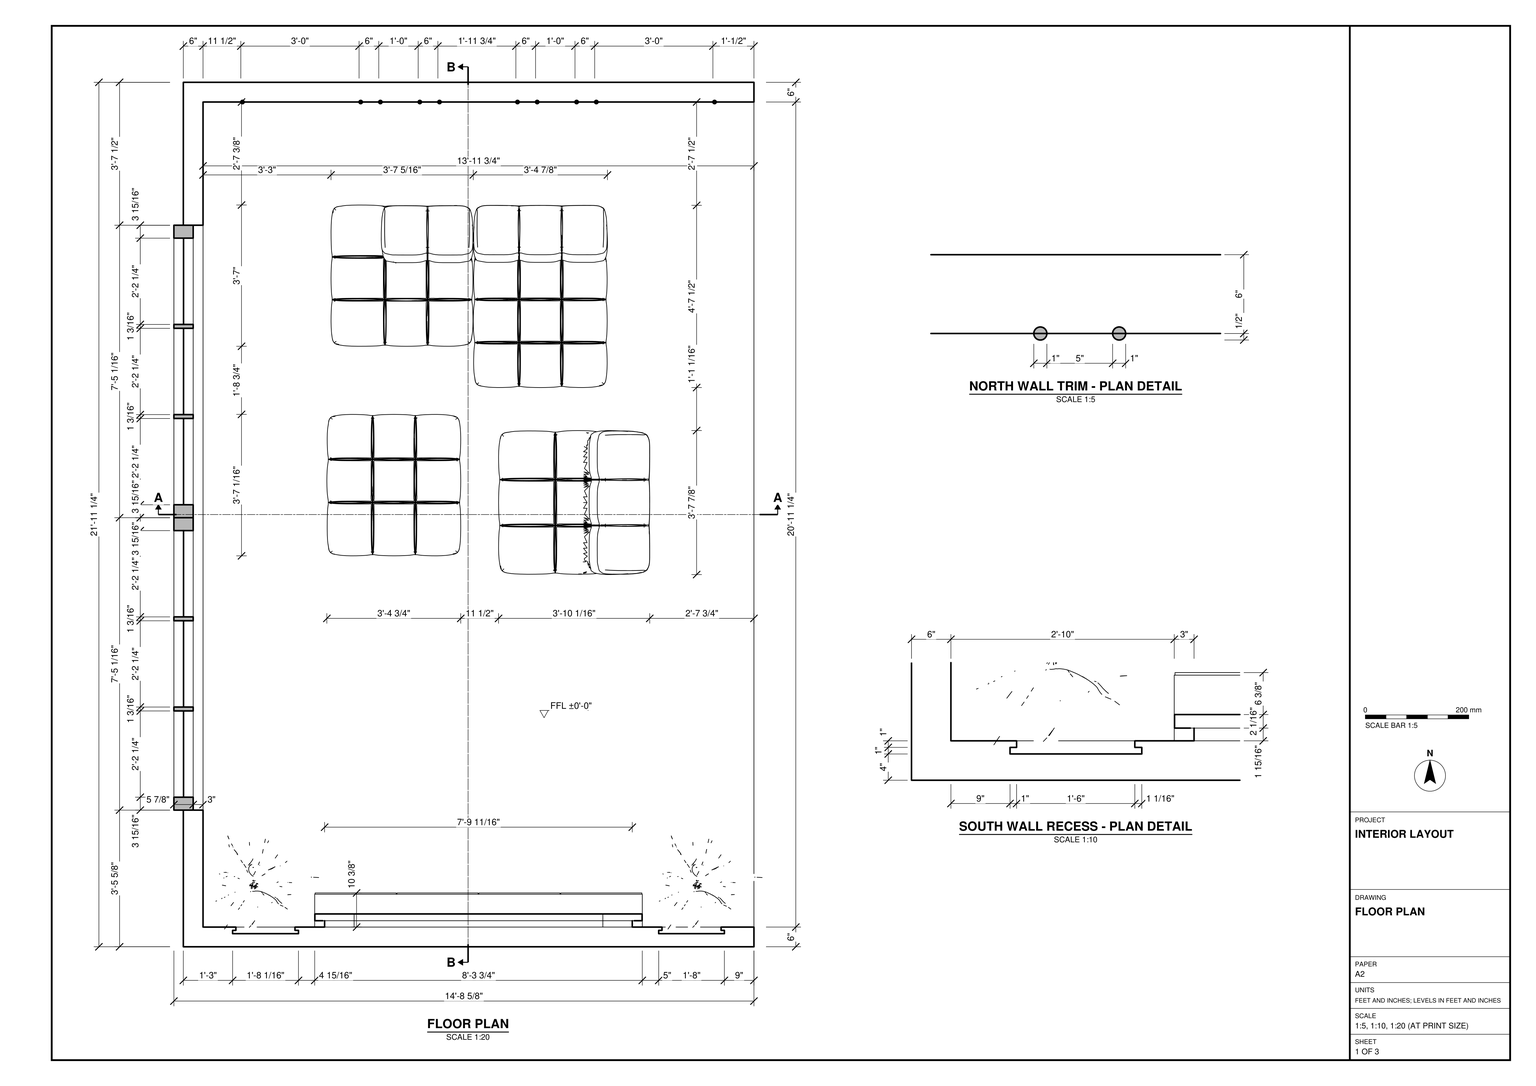
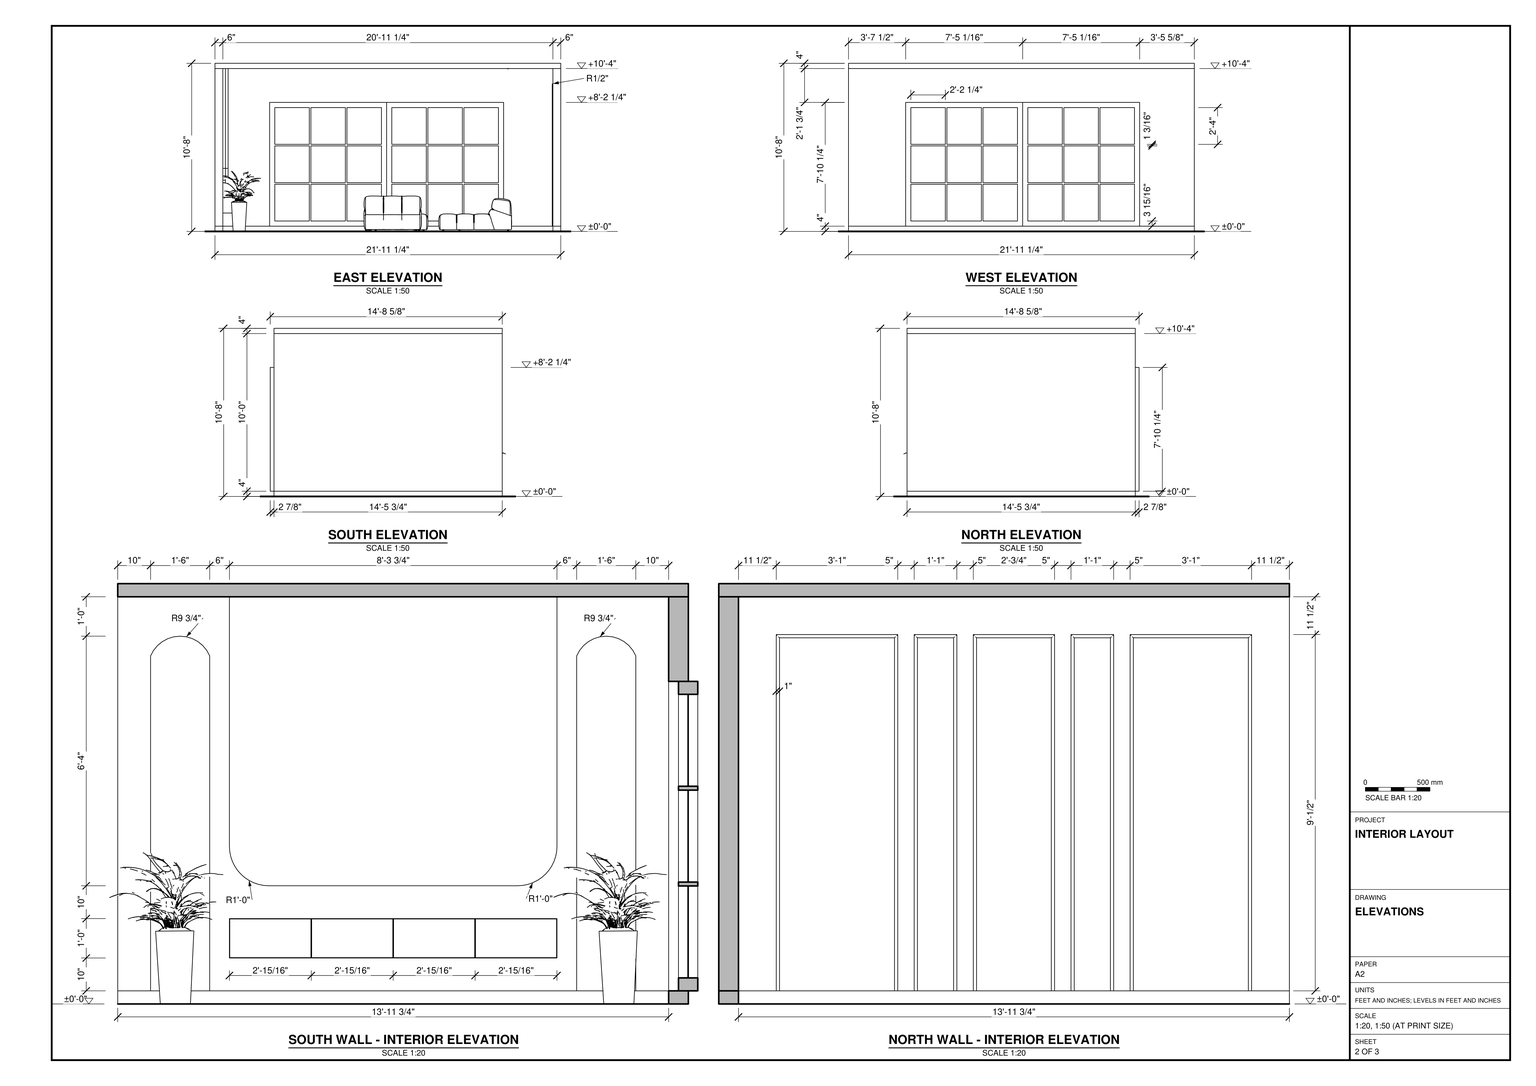
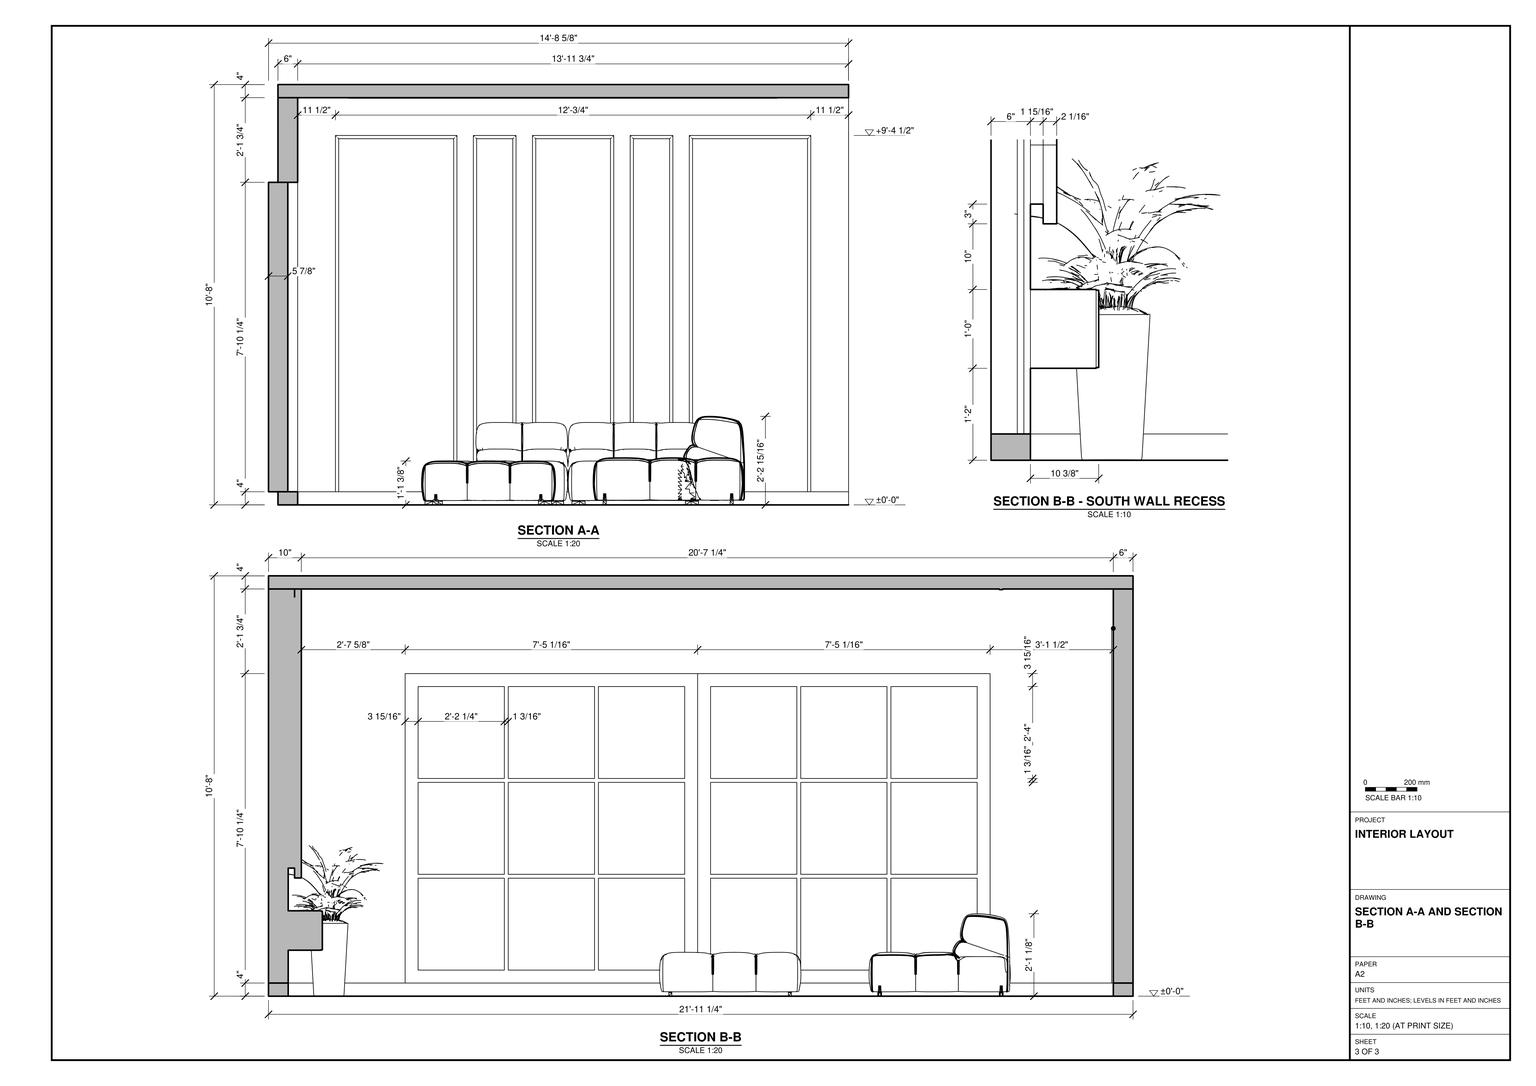
Build the lounge in SketchUp from task_files/diagram_01.pdf. Work in feet and inches. Use the floor plan to orient the room, with north at the top. The overall model extents are 14'-11 3/16" east to west, 21'-11 1/4" north to south and 10'-8" high. Use ±0'-0" as the single floor level.

Model the floor and ceiling slabs and the north, south and west walls with the thicknesses shown in plan and section. Leave the east side open as drawn. Fit the paired window units into the west wall, matching their frames and pane divisions. On the north wall, reproduce the tall rectangular trim outlines in their alternating widths. On the south wall, form the central panel with rounded lower corners, the arched recesses on either side and the floating four-front cabinet below the panel. Use the detail views to distinguish the recessed features from the projecting joinery.

Arrange the modular sofa toward the north wall with its deeper section on the east. Place the separate ottoman and backed seat to its south, matching their footprints and the gap between them. Decor and loose items, including the plants flanking the cabinet, may be any suitable library components, for example from 3D Warehouse. Keep shell elements and each furniture or joinery piece in separate groups or components, and use components for repeated parts. Save one SketchUp model as output_files/lounge_with_modular_seating_and_fitted_feature_walls.skp.

# SketchUp Ruby script. Lengths in inches.
U = 1.inch
M = Sketchup.active_model
def pt(a) = Geom::Point3d.new(a.map { |v| v * U })
def face(e, loops, mat)
  f = e.add_face(loops[0].map { |a| pt(a) })
  loops[1..].each { |l| e.add_face(l.map { |a| pt(a) }).erase! }
  f.material = f.back_material = mat if mat
  f
end
# faces: each face lists its corners as indices into pts; further lists are holes
def faces(e, pts, list, mat = nil) = list.each { |f| face(e, (f[0].is_a?(Array) ? f : [f]).map { |l| l.map { |i| pts[i] } }, mat) }
# xy, xz, yz: faces in a plane at the given z, y or x. An outline is a flat list of corners, or four numbers for a rectangle; further outlines are holes
def ring(l) = l.size == 4 ? [[l[0], l[1]], [l[2], l[1]], [l[2], l[3]], [l[0], l[3]]] : l.each_slice(2).to_a
def flat(e, list, mat, &to3) = list.each { |f| face(e, (f[0].is_a?(Array) ? f : [f]).map { |l| ring(l).map { |u, v| to3.(u, v) } }, mat) }
def xy(e, z, list, mat = nil) = flat(e, list, mat) { |x, y| [x, y, z] }
def xz(e, y, list, mat = nil) = flat(e, list, mat) { |x, z| [x, y, z] }
def yz(e, x, list, mat = nil) = flat(e, list, mat) { |y, z| [x, y, z] }
def lines(e, pts, list) = list.each { |a, b| e.add_line(pt(pts[a]), pt(pts[b])) }
# prism: a flat outline (further loops are holes) pulled along v
def prism(e, loops, v, mat = nil)
  f = face(e, loops, mat); d = Geom::Vector3d.new(v.map { |x| x * U })
  f.pushpull(f.normal.samedirection?(d) ? d.length : -d.length)
end
def box(e, o, s, mat = nil) = prism(e, [[o, [o[0] + s[0], o[1], o[2]], [o[0] + s[0], o[1] + s[1], o[2]], [o[0], o[1] + s[1], o[2]]]], [0, 0, s[2]], mat)
def at(x, y, z, deg = 0) = Geom::Transformation.translation(pt([x, y, z])) * Geom::Transformation.rotation(ORIGIN, Z_AXIS, deg.degrees)
def axes(o, x, y, z) = Geom::Transformation.new([*x, 0, *y, 0, *z, 0, *pt(o).to_a, 1])
def part(name) = M.definitions.add(name)
# library, detail: a bought-in or finely detailed component or shape, given as its bounding box
def library(name, o, s) = part(name).tap { |d| box(d.entities, o, s) }
def detail(e, o, s) = box(e.add_group.entities, o, s)
def put(e, d, t, mat = nil) = e.add_instance(d, t).tap { |i| i.material = mat if mat }
def group(e, t, mat = nil) = e.add_group.tap { |g| g.transformation = t; g.material = mat if mat }.entities
root = M.entities
M.materials.add("Emissive").color = [255, 255, 255]
M.materials.add("Generic").color = [218, 212, 201]
M.materials.add("Pine Matte 300cm").color = [173, 150, 115]
M.materials.add("Sandstone 150cm").color = [161, 146, 124]
M.materials.add("Stucco Shadow 300cm").color = [61, 59, 79]
M.materials.add("Sumele_Hair").color = [19, 13, 7]
M.materials.add("WALL P 1").color = [209, 201, 189]
M.materials.add("WALL P 2").color = [44, 39, 31]
M.materials.add("Wall Paint Dusk Blue Matte 300cm").color = [122, 143, 157]
M.materials.add("Wall Paint Olive Satin 300cm").color = [133, 140, 86]
M.materials.add("Wallpaper A04 Golden 40cm").color = [81, 64, 34]
M.materials.add("Walnut Matte 300cm").color = [111, 85, 55]
M.materials.add("[Metal Corrugated Shiny]").color = [193, 193, 193]
M.materials.add("[Translucent Glass Gray]").color = [128, 128, 128]
M.materials["[Translucent Glass Gray]"].alpha = 0.5
M.materials.add("sofa .").color = [225, 194, 69]
c1 = library("skpD0I6a8",[14.43,-68.68,0],[105.42,143.14,64.75])
c2 = library("skpcyxm1p",[14.43,-75.28,0],[105.19,111.11,34.48])
c3 = library("Modular lounge seating",[0,0,0],[105.41,111.76,64.75])
c4 = library("skp0QfVtK",[14.45,-36.06,-0.05],[111.77,111,64.8])
c5 = library("IES Light",[-4.45,-4.45,-12],[8.9,8.9,12])
c6 = part("Group30\#1")
p = [[0,0,0],[0,0,-64.71],[-12.88,0,-64.71],[83.875,-125.625,0],[-83.875,-125.625,0],[83.875,125.625,0],
  [83.875,0,0],[-83.875,125.625,0],[12.88,0,-64.71],[-83.875,0,0],[0,0,-104.75]]
lines(c6.entities,p,[[0,1],[1,2],[3,4],[5,6],[7,5],[1,8],[9,0],[0,6],[8,10],[4,9],[6,3],[2,10],
  [9,7]])
c7 = part("Rectangle Light")
put(c7.entities,c6,at(0,0,0))
c8 = library("Plant",[-15.17,-14.95,0],[35.27,31.45,46.14])
c9 = part("Group2\#2")
xy(c9.entities,0,[[-40.59,-43.18,-14.32,-15.18],[-13.13,-43.18,13.13,-15.18],[14.32,-43.18,40.59,-15.18],[-40.59,-14,-14.32,14],[-13.13,-14,13.13,14],
  [14.32,-14,40.59,14],[-40.59,15.18,-14.32,43.18],[-13.13,15.18,13.13,43.18],[14.32,15.18,40.59,43.18]])
c10 = part("Group1\#1")
prism(c10.entities,[[[44.53,47.11,0],[44.53,-47.11,0],[-44.53,-47.11,0],[-44.53,47.11,0]],[[-14.32,-43.18,0],[-14.32,-15.18,0],[-40.59,-15.18,0],[-40.59,-43.18,0]],[[-14.32,14,0],[-40.59,14,0],[-40.59,-14,0],[-14.32,-14,0]],[[-40.59,43.18,0],[-40.59,15.18,0],[-14.32,15.18,0],[-14.32,43.18,0]],[[14.32,-15.18,0],[14.32,-43.18,0],[40.59,-43.18,0],[40.59,-15.18,0]],[[-13.13,-43.18,0],[13.13,-43.18,0],[13.13,-15.18,0],[-13.13,-15.18,0]],[[13.13,15.18,0],[13.13,43.18,0],[-13.13,43.18,0],[-13.13,15.18,0]],[[14.32,15.18,0],[40.59,15.18,0],[40.59,43.18,0],[14.32,43.18,0]],[[-13.13,14,0],[-13.13,-14,0],[13.13,-14,0],[13.13,14,0]],[[14.32,14,0],[14.32,-14,0],[40.59,-14,0],[40.59,14,0]]],[0,0,5.875],"[Metal Corrugated Shiny]")
put(c10.entities,c9,at(0,0,2.9375),"[Translucent Glass Gray]")
c11 = part("Group4\#2")
xy(c11.entities,0,[[-40.59,-43.18,-14.32,-15.18],[-13.13,-43.18,13.13,-15.18],[14.32,-43.18,40.59,-15.18],[-40.59,-14,-14.32,14],[-13.13,-14,13.13,14],
  [14.32,-14,40.59,14],[-40.59,15.18,-14.32,43.18],[-13.13,15.18,13.13,43.18],[14.32,15.18,40.59,43.18]],"[Translucent Glass Gray]")
c12 = part("Group3\#1")
prism(c12.entities,[[[-44.53,-47.11,0],[-44.53,47.11,0],[44.53,47.11,0],[44.53,-47.11,0]],[[13.13,-15.18,0],[-13.13,-15.18,0],[-13.13,-43.18,0],[13.13,-43.18,0]],[[-13.13,14,0],[-13.13,-14,0],[13.13,-14,0],[13.13,14,0]],[[13.13,15.18,0],[13.13,43.18,0],[-13.13,43.18,0],[-13.13,15.18,0]],[[-40.59,14,0],[-40.59,-14,0],[-14.32,-14,0],[-14.32,14,0]],[[14.32,14,0],[14.32,-14,0],[40.59,-14,0],[40.59,14,0]],[[-40.59,-15.18,0],[-40.59,-43.18,0],[-14.32,-43.18,0],[-14.32,-15.18,0]],[[40.59,-43.18,0],[40.59,-15.18,0],[14.32,-15.18,0],[14.32,-43.18,0]],[[-40.59,43.18,0],[-40.59,15.18,0],[-14.32,15.18,0],[-14.32,43.18,0]],[[14.32,15.18,0],[40.59,15.18,0],[40.59,43.18,0],[14.32,43.18,0]]],[0,0,5.875],"[Metal Corrugated Shiny]")
put(c12.entities,c11,at(0,0,2.9375))
c13 = library("Group18\#1",[17.5,256.75,4],[144.75,1,108.5])
xy(root,0,[[2.875,0,176.625,0,176.625,6,8.875,6,8.875,257.25,176.625,257.25,176.625,263.25,2.875,263.25]])
xy(root,0,[[8.875,6,176.625,257.25]],"Generic")
xy(root,4,[[2.875,0,176.625,0,176.625,6,166.625,6,166.625,5,167.625,5,167.625,4,147.625,4,147.625,5,148.625,5,148.625,6,36.875,6,36.875,5,37.9375,5,37.9375,4,17.875,4,17.875,5,18.875,5,18.875,6,8.875,6,8.875,41.61,2.875,41.61],[17.875,4,37.9375,4,37.9375,5,36.875,5,36.875,6,18.875,6,18.875,5,17.875,5],[147.625,4,167.625,4,167.625,5,166.625,5,166.625,6,148.625,6,148.625,5,147.625,5],[2.875,41.61,5.875,219.73],[5.875,41.61,8.875,219.73],
  [2.875,219.73,8.875,219.73,8.875,257.25,176.625,257.25,176.625,263.25,2.875,263.25]])
xy(root,14,[[42.875,6,142.625,16]],"Pine Matte 300cm")
xy(root,14.12,[[42.99,16,67.69,16.39],[67.93,16,92.63,16.39],[92.87,16,117.57,16.39],[117.81,16,142.51,16.39]],"Walnut Matte 300cm")
xy(root,25.88,[[42.99,16,67.69,16.39],[67.93,16,92.63,16.39],[92.87,16,117.57,16.39],[117.81,16,142.51,16.39]],"Walnut Matte 300cm")
xy(root,26,[[42.875,6,142.625,16]],"Pine Matte 300cm")
xy(root,36,[[54.875,7.9375,130.625,10]],"Stucco Shadow 300cm")
xy(root,39,[[54.875,6,130.625,7.9375]],"Emissive")
xy(root,98.23,[[2.875,41.61,5.875,219.73],[5.875,41.61,8.875,219.73]])
xy(root,106,[[17.875,4,18.875,5],[36.875,4,37.9375,5],[147.625,4,148.625,5],[166.625,4,167.625,5]])
xy(root,123.8125,[[27.82,223.07,27.82,223.57,27.95,223.55,28.07,223.5,28.17,223.42,28.25,223.32,28.3,223.2,28.32,223.07],[142.32,223.07,142.32,223.57,142.45,223.55,142.57,223.5,142.67,223.42,142.75,223.32,142.8,223.2,142.82,223.07]])
xy(root,123.8125,[[27.82,222.57,27.69,222.58,27.57,222.63,27.47,222.71,27.39,222.82,27.34,222.9375,27.32,223.07,27.82,223.07],[27.82,222.57,27.82,223.07,28.32,223.07,28.3,222.9375,28.25,222.82,28.17,222.71,28.07,222.63,27.95,222.58],[29.82,222.57,29.69,222.58,29.57,222.63,29.47,222.71,29.39,222.82,29.34,222.9375,29.32,223.07,29.82,223.07],[29.82,222.57,29.82,223.07,30.32,223.07,30.3,222.9375,30.25,222.82,30.17,222.71,30.07,222.63,29.95,222.58],[31.82,222.57,31.69,222.58,31.57,222.63,31.47,222.71,31.39,222.82,31.34,222.9375,31.32,223.07,31.82,223.07],
  [31.82,222.57,31.82,223.07,32.32,223.07,32.3,222.9375,32.25,222.82,32.17,222.71,32.07,222.63,31.95,222.58],[33.82,222.57,33.69,222.58,33.57,222.63,33.47,222.71,33.39,222.82,33.34,222.9375,33.32,223.07,33.82,223.07],[33.82,222.57,33.82,223.07,34.32,223.07,34.3,222.9375,34.25,222.82,34.17,222.71,34.07,222.63,33.95,222.58],[35.82,222.57,35.69,222.58,35.57,222.63,35.47,222.71,35.39,222.82,35.34,222.9375,35.32,223.07,35.82,223.07],[35.82,222.57,35.82,223.07,36.32,223.07,36.3,222.9375,36.25,222.82,36.17,222.71,36.07,222.63,35.95,222.58],
  [67.51,222.57,67.38,222.58,67.26,222.63,67.15,222.71,67.07,222.82,67.02,222.9375,67.01,223.07,67.51,223.07],[67.51,222.57,67.51,223.07,68.01,223.07,67.99,222.9375,67.94,222.82,67.86,222.71,67.76,222.63,67.64,222.58],[69.51,222.57,69.38,222.58,69.26,222.63,69.15,222.71,69.07,222.82,69.02,222.9375,69.01,223.07,69.51,223.07],[69.51,222.57,69.51,223.07,70.01,223.07,69.99,222.9375,69.94,222.82,69.86,222.71,69.76,222.63,69.64,222.58],[71.51,222.57,71.38,222.58,71.26,222.63,71.15,222.71,71.07,222.82,71.02,222.9375,71.01,223.07,71.51,223.07],
  [71.51,222.57,71.51,223.07,72.01,223.07,71.99,222.9375,71.94,222.82,71.86,222.71,71.76,222.63,71.64,222.58],[73.51,222.57,73.38,222.58,73.26,222.63,73.15,222.71,73.07,222.82,73.02,222.9375,73.01,223.07,73.51,223.07],[73.51,222.57,73.51,223.07,74.01,223.07,73.99,222.9375,73.94,222.82,73.86,222.71,73.76,222.63,73.64,222.58],[75.51,222.57,75.38,222.58,75.26,222.63,75.15,222.71,75.07,222.82,75.02,222.9375,75.01,223.07,75.51,223.07],[75.51,222.57,75.51,223.07,76.01,223.07,75.99,222.9375,75.94,222.82,75.86,222.71,75.76,222.63,75.64,222.58],
  [107.07,222.57,106.94,222.58,106.82,222.63,106.72,222.71,106.64,222.82,106.59,222.9375,106.57,223.07,107.07,223.07],[107.07,222.57,107.07,223.07,107.57,223.07,107.55,222.9375,107.5,222.82,107.42,222.71,107.32,222.63,107.2,222.58],[109.07,222.57,108.94,222.58,108.82,222.63,108.72,222.71,108.64,222.82,108.59,222.9375,108.57,223.07,109.07,223.07],[109.07,222.57,109.07,223.07,109.57,223.07,109.55,222.9375,109.5,222.82,109.42,222.71,109.32,222.63,109.2,222.58],[111.07,222.57,110.94,222.58,110.82,222.63,110.72,222.71,110.64,222.82,110.59,222.9375,110.57,223.07,111.07,223.07],
  [111.07,222.57,111.07,223.07,111.57,223.07,111.55,222.9375,111.5,222.82,111.42,222.71,111.32,222.63,111.2,222.58],[113.07,222.57,112.94,222.58,112.82,222.63,112.72,222.71,112.64,222.82,112.59,222.9375,112.57,223.07,113.07,223.07],[113.07,222.57,113.07,223.07,113.57,223.07,113.55,222.9375,113.5,222.82,113.42,222.71,113.32,222.63,113.2,222.58],[115.07,222.57,114.94,222.58,114.82,222.63,114.72,222.71,114.64,222.82,114.59,222.9375,114.57,223.07,115.07,223.07],[115.07,222.57,115.07,223.07,115.57,223.07,115.55,222.9375,115.5,222.82,115.42,222.71,115.32,222.63,115.2,222.58],
  [138.32,222.57,138.19,222.58,138.07,222.63,137.97,222.71,137.89,222.82,137.84,222.9375,137.82,223.07,138.32,223.07],[138.32,222.57,138.32,223.07,138.82,223.07,138.8,222.9375,138.75,222.82,138.67,222.71,138.57,222.63,138.45,222.58],[140.32,222.57,140.19,222.58,140.07,222.63,139.97,222.71,139.89,222.82,139.84,222.9375,139.82,223.07,140.32,223.07],[140.32,222.57,140.32,223.07,140.82,223.07,140.8,222.9375,140.75,222.82,140.67,222.71,140.57,222.63,140.45,222.58],[142.32,222.57,142.19,222.58,142.07,222.63,141.97,222.71,141.89,222.82,141.84,222.9375,141.82,223.07,142.32,223.07],
  [142.32,222.57,142.32,223.07,142.82,223.07,142.8,222.9375,142.75,222.82,142.67,222.71,142.57,222.63,142.45,222.58],[144.32,222.57,144.19,222.58,144.07,222.63,143.97,222.71,143.89,222.82,143.84,222.9375,143.82,223.07,144.32,223.07],[144.32,222.57,144.32,223.07,144.82,223.07,144.8,222.9375,144.75,222.82,144.67,222.71,144.57,222.63,144.45,222.58],[146.32,222.57,146.19,222.58,146.07,222.63,145.97,222.71,145.89,222.82,145.84,222.9375,145.82,223.07,146.32,223.07],[146.32,222.57,146.32,223.07,146.82,223.07,146.8,222.9375,146.75,222.82,146.67,222.71,146.57,222.63,146.45,222.58],
  [27.32,223.07,27.34,223.2,27.39,223.32,27.47,223.42,27.57,223.5,27.69,223.55,27.82,223.57,27.82,223.07],[29.32,223.07,29.34,223.2,29.39,223.32,29.47,223.42,29.57,223.5,29.69,223.55,29.82,223.57,29.82,223.07],[29.82,223.07,29.82,223.57,29.95,223.55,30.07,223.5,30.17,223.42,30.25,223.32,30.3,223.2,30.32,223.07],[31.32,223.07,31.34,223.2,31.39,223.32,31.47,223.42,31.57,223.5,31.69,223.55,31.82,223.57,31.82,223.07],[31.82,223.07,31.82,223.57,31.95,223.55,32.07,223.5,32.17,223.42,32.25,223.32,32.3,223.2,32.32,223.07],
  [33.32,223.07,33.34,223.2,33.39,223.32,33.47,223.42,33.57,223.5,33.69,223.55,33.82,223.57,33.82,223.07],[33.82,223.07,33.82,223.57,33.95,223.55,34.07,223.5,34.17,223.42,34.25,223.32,34.3,223.2,34.32,223.07],[35.32,223.07,35.34,223.2,35.39,223.32,35.47,223.42,35.57,223.5,35.69,223.55,35.82,223.57,35.82,223.07],[35.82,223.07,35.82,223.57,35.95,223.55,36.07,223.5,36.17,223.42,36.25,223.32,36.3,223.2,36.32,223.07],[67.01,223.07,67.02,223.2,67.07,223.32,67.15,223.42,67.26,223.5,67.38,223.55,67.51,223.57,67.51,223.07],
  [67.51,223.07,67.51,223.57,67.64,223.55,67.76,223.5,67.86,223.42,67.94,223.32,67.99,223.2,68.01,223.07],[69.01,223.07,69.02,223.2,69.07,223.32,69.15,223.42,69.26,223.5,69.38,223.55,69.51,223.57,69.51,223.07],[69.51,223.07,69.51,223.57,69.64,223.55,69.76,223.5,69.86,223.42,69.94,223.32,69.99,223.2,70.01,223.07],[71.01,223.07,71.02,223.2,71.07,223.32,71.15,223.42,71.26,223.5,71.38,223.55,71.51,223.57,71.51,223.07],[71.51,223.07,71.51,223.57,71.64,223.55,71.76,223.5,71.86,223.42,71.94,223.32,71.99,223.2,72.01,223.07],
  [73.01,223.07,73.02,223.2,73.07,223.32,73.15,223.42,73.26,223.5,73.38,223.55,73.51,223.57,73.51,223.07],[73.51,223.07,73.51,223.57,73.64,223.55,73.76,223.5,73.86,223.42,73.94,223.32,73.99,223.2,74.01,223.07],[75.01,223.07,75.02,223.2,75.07,223.32,75.15,223.42,75.26,223.5,75.38,223.55,75.51,223.57,75.51,223.07],[75.51,223.07,75.51,223.57,75.64,223.55,75.76,223.5,75.86,223.42,75.94,223.32,75.99,223.2,76.01,223.07],[106.57,223.07,106.59,223.2,106.64,223.32,106.72,223.42,106.82,223.5,106.94,223.55,107.07,223.57,107.07,223.07],
  [107.07,223.07,107.07,223.57,107.2,223.55,107.32,223.5,107.42,223.42,107.5,223.32,107.55,223.2,107.57,223.07],[108.57,223.07,108.59,223.2,108.64,223.32,108.72,223.42,108.82,223.5,108.94,223.55,109.07,223.57,109.07,223.07],[109.07,223.07,109.07,223.57,109.2,223.55,109.32,223.5,109.42,223.42,109.5,223.32,109.55,223.2,109.57,223.07],[110.57,223.07,110.59,223.2,110.64,223.32,110.72,223.42,110.82,223.5,110.94,223.55,111.07,223.57,111.07,223.07],[111.07,223.07,111.07,223.57,111.2,223.55,111.32,223.5,111.42,223.42,111.5,223.32,111.55,223.2,111.57,223.07],
  [112.57,223.07,112.59,223.2,112.64,223.32,112.72,223.42,112.82,223.5,112.94,223.55,113.07,223.57,113.07,223.07],[113.07,223.07,113.07,223.57,113.2,223.55,113.32,223.5,113.42,223.42,113.5,223.32,113.55,223.2,113.57,223.07],[114.57,223.07,114.59,223.2,114.64,223.32,114.72,223.42,114.82,223.5,114.94,223.55,115.07,223.57,115.07,223.07],[115.07,223.07,115.07,223.57,115.2,223.55,115.32,223.5,115.42,223.42,115.5,223.32,115.55,223.2,115.57,223.07],[137.82,223.07,137.84,223.2,137.89,223.32,137.97,223.42,138.07,223.5,138.19,223.55,138.32,223.57,138.32,223.07],
  [138.32,223.07,138.32,223.57,138.45,223.55,138.57,223.5,138.67,223.42,138.75,223.32,138.8,223.2,138.82,223.07],[139.82,223.07,139.84,223.2,139.89,223.32,139.97,223.42,140.07,223.5,140.19,223.55,140.32,223.57,140.32,223.07],[140.32,223.07,140.32,223.57,140.45,223.55,140.57,223.5,140.67,223.42,140.75,223.32,140.8,223.2,140.82,223.07],[141.82,223.07,141.84,223.2,141.89,223.32,141.97,223.42,142.07,223.5,142.19,223.55,142.32,223.57,142.32,223.07],[143.82,223.07,143.84,223.2,143.89,223.32,143.97,223.42,144.07,223.5,144.19,223.55,144.32,223.57,144.32,223.07],
  [144.32,223.07,144.32,223.57,144.45,223.55,144.57,223.5,144.67,223.42,144.75,223.32,144.8,223.2,144.82,223.07],[145.82,223.07,145.84,223.2,145.89,223.32,145.97,223.42,146.07,223.5,146.19,223.55,146.32,223.57,146.32,223.07],[146.32,223.07,146.32,223.57,146.45,223.55,146.57,223.5,146.67,223.42,146.75,223.32,146.8,223.2,146.82,223.07]],"Emissive")
xy(root,123.8125,[[24.41,222.57,24.41,223.07,27.32,223.07,27.34,222.9375,27.39,222.82,27.47,222.71,27.57,222.63,27.69,222.58,27.82,222.57],[27.82,222.57,27.95,222.58,28.07,222.63,28.17,222.71,28.25,222.82,28.3,222.9375,28.32,223.07,29.32,223.07,29.34,222.9375,29.39,222.82,29.47,222.71,29.57,222.63,29.69,222.58,29.82,222.57],[29.82,222.57,29.95,222.58,30.07,222.63,30.17,222.71,30.25,222.82,30.3,222.9375,30.32,223.07,31.32,223.07,31.34,222.9375,31.39,222.82,31.47,222.71,31.57,222.63,31.69,222.58,31.82,222.57],[31.82,222.57,31.95,222.58,32.07,222.63,32.17,222.71,32.25,222.82,32.3,222.9375,32.32,223.07,33.32,223.07,33.34,222.9375,33.39,222.82,33.47,222.71,33.57,222.63,33.69,222.58,33.82,222.57],[33.82,222.57,33.95,222.58,34.07,222.63,34.17,222.71,34.25,222.82,34.3,222.9375,34.32,223.07,35.32,223.07,35.34,222.9375,35.39,222.82,35.47,222.71,35.57,222.63,35.69,222.58,35.82,222.57],
  [35.82,222.57,35.95,222.58,36.07,222.63,36.17,222.71,36.25,222.82,36.3,222.9375,36.32,223.07,67.01,223.07,67.02,222.9375,67.07,222.82,67.15,222.71,67.26,222.63,67.38,222.58,67.51,222.57],[67.51,222.57,67.64,222.58,67.76,222.63,67.86,222.71,67.94,222.82,67.99,222.9375,68.01,223.07,69.01,223.07,69.02,222.9375,69.07,222.82,69.15,222.71,69.26,222.63,69.38,222.58,69.51,222.57],[69.51,222.57,69.64,222.58,69.76,222.63,69.86,222.71,69.94,222.82,69.99,222.9375,70.01,223.07,71.01,223.07,71.02,222.9375,71.07,222.82,71.15,222.71,71.26,222.63,71.38,222.58,71.51,222.57],[71.51,222.57,71.64,222.58,71.76,222.63,71.86,222.71,71.94,222.82,71.99,222.9375,72.01,223.07,73.01,223.07,73.02,222.9375,73.07,222.82,73.15,222.71,73.26,222.63,73.38,222.58,73.51,222.57],[73.51,222.57,73.64,222.58,73.76,222.63,73.86,222.71,73.94,222.82,73.99,222.9375,74.01,223.07,75.01,223.07,75.02,222.9375,75.07,222.82,75.15,222.71,75.26,222.63,75.38,222.58,75.51,222.57],
  [75.51,222.57,75.64,222.58,75.76,222.63,75.86,222.71,75.94,222.82,75.99,222.9375,76.01,223.07,106.57,223.07,106.59,222.9375,106.64,222.82,106.72,222.71,106.82,222.63,106.94,222.58,107.07,222.57],[107.07,222.57,107.2,222.58,107.32,222.63,107.42,222.71,107.5,222.82,107.55,222.9375,107.57,223.07,108.57,223.07,108.59,222.9375,108.64,222.82,108.72,222.71,108.82,222.63,108.94,222.58,109.07,222.57],[109.07,222.57,109.2,222.58,109.32,222.63,109.42,222.71,109.5,222.82,109.55,222.9375,109.57,223.07,110.57,223.07,110.59,222.9375,110.64,222.82,110.72,222.71,110.82,222.63,110.94,222.58,111.07,222.57],[111.07,222.57,111.2,222.58,111.32,222.63,111.42,222.71,111.5,222.82,111.55,222.9375,111.57,223.07,112.57,223.07,112.59,222.9375,112.64,222.82,112.72,222.71,112.82,222.63,112.94,222.58,113.07,222.57],[113.07,222.57,113.2,222.58,113.32,222.63,113.42,222.71,113.5,222.82,113.55,222.9375,113.57,223.07,114.57,223.07,114.59,222.9375,114.64,222.82,114.72,222.71,114.82,222.63,114.94,222.58,115.07,222.57],
  [115.07,222.57,115.2,222.58,115.32,222.63,115.42,222.71,115.5,222.82,115.55,222.9375,115.57,223.07,137.82,223.07,137.84,222.9375,137.89,222.82,137.97,222.71,138.07,222.63,138.19,222.58,138.32,222.57],[138.32,222.57,138.45,222.58,138.57,222.63,138.67,222.71,138.75,222.82,138.8,222.9375,138.82,223.07,139.82,223.07,139.84,222.9375,139.89,222.82,139.97,222.71,140.07,222.63,140.19,222.58,140.32,222.57],[140.32,222.57,140.45,222.58,140.57,222.63,140.67,222.71,140.75,222.82,140.8,222.9375,140.82,223.07,141.82,223.07,141.84,222.9375,141.89,222.82,141.97,222.71,142.07,222.63,142.19,222.58,142.32,222.57],[142.32,222.57,142.45,222.58,142.57,222.63,142.67,222.71,142.75,222.82,142.8,222.9375,142.82,223.07,143.82,223.07,143.84,222.9375,143.89,222.82,143.97,222.71,144.07,222.63,144.19,222.58,144.32,222.57],[144.32,222.57,144.45,222.58,144.57,222.63,144.67,222.71,144.75,222.82,144.8,222.9375,144.82,223.07,145.82,223.07,145.84,222.9375,145.89,222.82,145.97,222.71,146.07,222.63,146.19,222.58,146.32,222.57],
  [146.32,222.57,146.45,222.58,146.57,222.63,146.67,222.71,146.75,222.82,146.8,222.9375,146.82,223.07,154.91,223.07,154.91,222.57],[24.41,223.07,24.41,223.57,27.82,223.57,27.69,223.55,27.57,223.5,27.47,223.42,27.39,223.32,27.34,223.2,27.32,223.07],[28.32,223.07,28.3,223.2,28.25,223.32,28.17,223.42,28.07,223.5,27.95,223.55,27.82,223.57,29.82,223.57,29.69,223.55,29.57,223.5,29.47,223.42,29.39,223.32,29.34,223.2,29.32,223.07],[30.32,223.07,30.3,223.2,30.25,223.32,30.17,223.42,30.07,223.5,29.95,223.55,29.82,223.57,31.82,223.57,31.69,223.55,31.57,223.5,31.47,223.42,31.39,223.32,31.34,223.2,31.32,223.07],[32.32,223.07,32.3,223.2,32.25,223.32,32.17,223.42,32.07,223.5,31.95,223.55,31.82,223.57,33.82,223.57,33.69,223.55,33.57,223.5,33.47,223.42,33.39,223.32,33.34,223.2,33.32,223.07],
  [34.32,223.07,34.3,223.2,34.25,223.32,34.17,223.42,34.07,223.5,33.95,223.55,33.82,223.57,35.82,223.57,35.69,223.55,35.57,223.5,35.47,223.42,35.39,223.32,35.34,223.2,35.32,223.07],[36.32,223.07,36.3,223.2,36.25,223.32,36.17,223.42,36.07,223.5,35.95,223.55,35.82,223.57,67.51,223.57,67.38,223.55,67.26,223.5,67.15,223.42,67.07,223.32,67.02,223.2,67.01,223.07],[68.01,223.07,67.99,223.2,67.94,223.32,67.86,223.42,67.76,223.5,67.64,223.55,67.51,223.57,69.51,223.57,69.38,223.55,69.26,223.5,69.15,223.42,69.07,223.32,69.02,223.2,69.01,223.07],[70.01,223.07,69.99,223.2,69.94,223.32,69.86,223.42,69.76,223.5,69.64,223.55,69.51,223.57,71.51,223.57,71.38,223.55,71.26,223.5,71.15,223.42,71.07,223.32,71.02,223.2,71.01,223.07],[72.01,223.07,71.99,223.2,71.94,223.32,71.86,223.42,71.76,223.5,71.64,223.55,71.51,223.57,73.51,223.57,73.38,223.55,73.26,223.5,73.15,223.42,73.07,223.32,73.02,223.2,73.01,223.07],
  [74.01,223.07,73.99,223.2,73.94,223.32,73.86,223.42,73.76,223.5,73.64,223.55,73.51,223.57,75.51,223.57,75.38,223.55,75.26,223.5,75.15,223.42,75.07,223.32,75.02,223.2,75.01,223.07],[76.01,223.07,75.99,223.2,75.94,223.32,75.86,223.42,75.76,223.5,75.64,223.55,75.51,223.57,107.07,223.57,106.94,223.55,106.82,223.5,106.72,223.42,106.64,223.32,106.59,223.2,106.57,223.07],[107.57,223.07,107.55,223.2,107.5,223.32,107.42,223.42,107.32,223.5,107.2,223.55,107.07,223.57,109.07,223.57,108.94,223.55,108.82,223.5,108.72,223.42,108.64,223.32,108.59,223.2,108.57,223.07],[109.57,223.07,109.55,223.2,109.5,223.32,109.42,223.42,109.32,223.5,109.2,223.55,109.07,223.57,111.07,223.57,110.94,223.55,110.82,223.5,110.72,223.42,110.64,223.32,110.59,223.2,110.57,223.07],[111.57,223.07,111.55,223.2,111.5,223.32,111.42,223.42,111.32,223.5,111.2,223.55,111.07,223.57,113.07,223.57,112.94,223.55,112.82,223.5,112.72,223.42,112.64,223.32,112.59,223.2,112.57,223.07],
  [113.57,223.07,113.55,223.2,113.5,223.32,113.42,223.42,113.32,223.5,113.2,223.55,113.07,223.57,115.07,223.57,114.94,223.55,114.82,223.5,114.72,223.42,114.64,223.32,114.59,223.2,114.57,223.07],[115.57,223.07,115.55,223.2,115.5,223.32,115.42,223.42,115.32,223.5,115.2,223.55,115.07,223.57,138.32,223.57,138.19,223.55,138.07,223.5,137.97,223.42,137.89,223.32,137.84,223.2,137.82,223.07],[138.82,223.07,138.8,223.2,138.75,223.32,138.67,223.42,138.57,223.5,138.45,223.55,138.32,223.57,140.32,223.57,140.19,223.55,140.07,223.5,139.97,223.42,139.89,223.32,139.84,223.2,139.82,223.07],[140.82,223.07,140.8,223.2,140.75,223.32,140.67,223.42,140.57,223.5,140.45,223.55,140.32,223.57,142.32,223.57,142.19,223.55,142.07,223.5,141.97,223.42,141.89,223.32,141.84,223.2,141.82,223.07],[142.82,223.07,142.8,223.2,142.75,223.32,142.67,223.42,142.57,223.5,142.45,223.55,142.32,223.57,144.32,223.57,144.19,223.55,144.07,223.5,143.97,223.42,143.89,223.32,143.84,223.2,143.82,223.07],
  [144.82,223.07,144.8,223.2,144.75,223.32,144.67,223.42,144.57,223.5,144.45,223.55,144.32,223.57,146.32,223.57,146.19,223.55,146.07,223.5,145.97,223.42,145.89,223.32,145.84,223.2,145.82,223.07],[146.82,223.07,146.8,223.2,146.75,223.32,146.67,223.42,146.57,223.5,146.45,223.55,146.32,223.57,154.91,223.57,154.91,223.07]],"Sumele_Hair")
xy(root,124,[[2.875,0,176.625,0,176.625,6,8.875,6,8.875,257.25,176.625,257.25,176.625,263.25,2.875,263.25],[[8.875,6,8.875,257.25,176.625,257.25,176.625,6,139.625,6,139.625,7.9375,142.625,7.9375,142.625,10,42.875,10,42.875,7.9375,45.875,7.9375,45.875,6],[24.41,222.57,154.91,223.57]],[45.875,6,139.625,7.9375],[42.875,7.9375,142.625,10],[42.875,7.9375,142.625,10]])
xy(root,128,[[2.875,0,176.625,263.25]])
xz(root,0,[[2.875,0,176.625,4],[2.875,4,176.625,124],[2.875,124,176.625,128]])
xz(root,4,[[17.875,4,17.875,106,18.875,106,19.78,107.68,20.99,109.15,22.47,110.36,24.15,111.26,25.98,111.8125,27.875,112,29.77,111.8125,31.6,111.26,33.28,110.36,34.76,109.15,35.97,107.68,36.875,106,37.9375,106,37.9375,4],[147.625,4,147.625,106,148.625,106,149.53,107.68,150.74,109.15,152.22,110.36,153.9,111.26,155.73,111.8125,157.625,112,159.52,111.8125,161.35,111.26,163.03,110.36,164.51,109.15,165.72,107.68,166.625,106,167.625,106,167.625,4]],"Wallpaper A04 Golden 40cm")
xz(root,5,[[17.875,4,18.875,106],[36.875,4,37.9375,106],[147.625,4,148.625,106],[166.625,4,167.625,106]])
xz(root,6,[[8.875,0,176.625,4]])
xz(root,6,[[[8.875,4,8.875,124,45.875,124,45.875,48,45.9,46.81,46.09,45.63,46.45,44.49,46.95,43.41,47.6,42.41,48.39,41.51,49.29,40.73,50.29,40.08,51.37,39.57,52.51,39.22,53.68,39.03,54.875,39,130.625,39,131.8,39.08,132.95,39.31,134.07,39.69,135.125,40.21,136.1,40.86,136.99,41.64,137.77,42.52,138.42,43.5,138.94,44.56,139.32,45.67,139.55,46.83,139.625,48,139.625,124,176.625,124,176.625,4,166.625,4,166.625,106,165.72,107.68,164.51,109.15,163.03,110.36,161.35,111.26,159.52,111.8125,157.625,112,155.73,111.8125,153.9,111.26,152.22,110.36,150.74,109.15,149.53,107.68,148.625,106,148.625,4,36.875,4,36.875,106,35.97,107.68,34.76,109.15,33.28,110.36,31.6,111.26,29.77,111.8125,27.875,112,25.98,111.8125,24.15,111.26,22.47,110.36,20.99,109.15,19.78,107.68,18.875,106,18.875,4],[42.875,14,142.625,26]]],"Sandstone 150cm")
xz(root,7.9375,[[54.875,36,53.31,36.1,51.77,36.41,50.28,36.91,48.875,37.61,47.57,38.48,46.39,39.51,45.35,40.69,44.48,42,43.79,43.41,43.28,44.89,42.98,46.43,42.875,48,45.29,48,45.37,46.75,45.61,45.52,46.02,44.33,46.57,43.21,47.27,42.16,48.1,41.22,49.04,40.39,50.08,39.7,51.21,39.14,52.39,38.74,53.625,38.5,54.875,38.41],[54.875,36,130.625,38.41],[130.625,36,132.19,36.1,133.73,36.41,135.22,36.91,136.625,37.61,137.93,38.48,139.11,39.51,140.15,40.69,141.02,42,141.71,43.41,142.22,44.89,142.52,46.43,142.625,48,140.21,48,140.13,46.75,139.89,45.52,139.48,44.33,138.93,43.21,138.23,42.16,137.4,41.22,136.46,40.39,135.42,39.7,134.29,39.14,133.11,38.74,131.875,38.5,130.625,38.41],[54.875,38.41,130.625,39],[42.875,48,45.29,48,45.29,121.59,45.875,121.59,45.875,124,42.875,124],
  [45.29,48,45.875,121.59],[139.625,48,140.21,121.59],[140.21,48,142.625,48,142.625,124,139.625,124,139.625,121.59,140.21,121.59],[45.875,121.59,139.625,124]])
xz(root,10,[[54.875,36,53.31,36.1,51.77,36.41,50.28,36.91,48.875,37.61,47.57,38.48,46.39,39.51,45.35,40.69,44.48,42,43.79,43.41,43.28,44.89,42.98,46.43,42.875,48,42.875,124,142.625,124,142.625,48,142.52,46.43,142.22,44.89,141.71,43.41,141.02,42,140.15,40.69,139.11,39.51,137.93,38.48,136.625,37.61,135.22,36.91,133.73,36.41,132.19,36.1,130.625,36]],"Stucco Shadow 300cm")
xz(root,16,[[[42.875,14,67.8125,26],[42.99,14.12,67.69,25.88]],[[67.8125,14,92.75,26],[67.93,14.12,92.63,25.88]],[[92.75,14,117.6875,26],[92.87,14.12,117.57,25.88]],[[117.6875,14,142.625,26],[117.81,14.12,142.51,25.88]]],"Pine Matte 300cm")
xz(root,16.39,[[42.99,14.12,67.69,25.88],[67.93,14.12,92.63,25.88],[92.87,14.12,117.57,25.88],[117.81,14.12,142.51,25.88]],"Walnut Matte 300cm")
xz(root,41.61,[[2.875,4,5.875,98.23],[5.875,4,8.875,98.23]])
xz(root,219.73,[[2.875,4,5.875,98.23],[5.875,4,8.875,98.23]])
xz(root,222.57,[[24.41,123.8125,154.91,124]])
xz(root,223.57,[[24.41,123.8125,154.91,124]])
xz(root,257.25,[[8.875,0,176.625,4]])
xz(root,257.25,[[8.875,4,20.875,4,20.875,112,56.875,112,56.875,4,62.875,4,62.875,112,74.875,112,74.875,4,80.875,4,80.875,112,104.625,112,104.625,4,110.625,4,110.625,112,122.625,112,122.625,4,128.625,4,128.625,112,164.625,112,164.625,4,176.625,4,176.625,124,8.875,124]],"Sandstone 150cm")
xz(root,257.25,[[20.875,4,56.875,112],[128.625,4,164.625,112]],"WALL P 1")
xz(root,257.25,[[62.875,4,74.875,112],[110.625,4,122.625,112]],"WALL P 2")
xz(root,257.25,[[80.875,4,104.625,112]],"Wall Paint Dusk Blue Matte 300cm")
xz(root,263.25,[[2.875,0,176.625,4],[2.875,4,176.625,124],[2.875,124,176.625,128]])
yz(root,2.875,[[0,0,263.25,4],[0,4,0,124,263.25,124,263.25,4,219.73,4,219.73,98.23,41.61,98.23,41.61,4],[0,124,263.25,128]])
yz(root,8.875,[[6,0,257.25,4]])
yz(root,8.875,[[6,4,41.61,4,41.61,98.23,219.73,98.23,219.73,4,257.25,4,257.25,124,6,124]],"Wall Paint Olive Satin 300cm")
yz(root,17.875,[[4,4,5,106]],"Emissive")
yz(root,18.875,[[5,4,6,106]],"Sandstone 150cm")
yz(root,24.41,[[222.57,123.8125,223.57,124]])
yz(root,36.875,[[5,4,6,106]],"Sandstone 150cm")
yz(root,37.9375,[[4,4,5,106]],"Emissive")
yz(root,42.875,[[6,14,16,26]],"Pine Matte 300cm")
yz(root,42.875,[[7.9375,48,10,124]],"Stucco Shadow 300cm")
yz(root,42.99,[[16,14.12,16.39,25.88]],"Walnut Matte 300cm")
yz(root,45.875,[[6,48,7.9375,124]],"Emissive")
yz(root,67.69,[[16,14.12,16.39,25.88]],"Walnut Matte 300cm")
yz(root,67.93,[[16,14.12,16.39,25.88]],"Walnut Matte 300cm")
yz(root,92.63,[[16,14.12,16.39,25.88]],"Walnut Matte 300cm")
yz(root,92.87,[[16,14.12,16.39,25.88]],"Walnut Matte 300cm")
yz(root,117.57,[[16,14.12,16.39,25.88]],"Walnut Matte 300cm")
yz(root,117.81,[[16,14.12,16.39,25.88]],"Walnut Matte 300cm")
yz(root,139.625,[[6,48,7.9375,124]],"Emissive")
yz(root,142.51,[[16,14.12,16.39,25.88]])
yz(root,142.625,[[6,14,16,26]],"Pine Matte 300cm")
yz(root,142.625,[[7.9375,48,10,124]],"Stucco Shadow 300cm")
yz(root,147.625,[[4,4,5,106]],"Emissive")
yz(root,148.625,[[5,4,6,106]],"Sandstone 150cm")
yz(root,154.91,[[222.57,123.8125,223.57,124]])
yz(root,166.625,[[5,4,6,106]],"Sandstone 150cm")
yz(root,167.625,[[4,4,5,106]],"Emissive")
yz(root,176.625,[[0,0,6,4],[257.25,0,263.25,4],[0,4,6,124],[257.25,4,263.25,124],[0,124,263.25,128]])
p = [[53.31,10,36.1],[54.875,10,36],[54.875,7.9375,36],[53.31,7.9375,36.1],[130.625,10,36],[132.19,10,36.1],
  [132.19,7.9375,36.1],[130.625,7.9375,36],[51.77,10,36.41],[51.77,7.9375,36.41],[133.73,10,36.41],[133.73,7.9375,36.41],
  [50.28,10,36.91],[50.28,7.9375,36.91],[135.22,10,36.91],[135.22,7.9375,36.91],[48.875,10,37.61],[48.875,7.9375,37.61],
  [136.625,10,37.61],[136.625,7.9375,37.61],[47.57,10,38.48],[47.57,7.9375,38.48],[137.93,10,38.48],[137.93,7.9375,38.48],
  [46.39,10,39.51],[46.39,7.9375,39.51],[139.11,10,39.51],[139.11,7.9375,39.51],[53.68,6,39.03],[52.51,6,39.22],
  [52.51,7.9375,39.22],[53.68,7.9375,39.03],[54.875,6,39],[54.875,7.9375,39],[131.8,6,39.08],[130.625,6,39],
  [130.625,7.9375,39],[131.8,7.9375,39.08],[132.95,6,39.31],[132.95,7.9375,39.31],[51.37,6,39.57],[51.37,7.9375,39.57],
  [134.07,6,39.69],[134.07,7.9375,39.69],[45.35,10,40.69],[45.35,7.9375,40.69],[140.15,10,40.69],[140.15,7.9375,40.69],
  [50.29,6,40.08],[50.29,7.9375,40.08],[135.125,6,40.21],[135.125,7.9375,40.21],[49.29,6,40.73],[49.29,7.9375,40.73],
  [136.1,6,40.86],[136.1,7.9375,40.86],[48.39,6,41.51],[48.39,7.9375,41.51],[44.48,10,42],[44.48,7.9375,42],
  [141.02,10,42],[141.02,7.9375,42],[136.99,6,41.64],[136.99,7.9375,41.64],[47.6,6,42.41],[47.6,7.9375,42.41],
  [137.77,6,42.52],[137.77,7.9375,42.52],[43.79,10,43.41],[43.79,7.9375,43.41],[141.71,10,43.41],[141.71,7.9375,43.41],
  [46.95,6,43.41],[46.95,7.9375,43.41],[138.42,6,43.5],[138.42,7.9375,43.5],[46.45,6,44.49],[46.45,7.9375,44.49],
  [43.28,10,44.89],[43.28,7.9375,44.89],[142.22,10,44.89],[142.22,7.9375,44.89],[138.94,6,44.56],[138.94,7.9375,44.56],
  [46.09,6,45.63],[46.09,7.9375,45.63],[139.32,6,45.67],[139.32,7.9375,45.67],[42.98,10,46.43],[42.98,7.9375,46.43],
  [142.52,10,46.43],[142.52,7.9375,46.43],[45.9,6,46.81],[45.9,7.9375,46.81],[139.55,6,46.83],[139.55,7.9375,46.83],
  [42.875,10,48],[42.875,7.9375,48],[142.625,10,48],[142.625,7.9375,48],[45.875,6,48],[45.875,7.9375,48],
  [139.625,6,48],[139.625,7.9375,48],[18.875,6,106],[19.78,6,107.68],[19.78,4,107.68],[18.875,4,106],
  [18.875,5,106],[35.97,6,107.68],[36.875,6,106],[36.875,5,106],[36.875,4,106],[35.97,4,107.68],
  [148.625,6,106],[149.53,6,107.68],[149.53,4,107.68],[148.625,4,106],[148.625,5,106],[165.72,6,107.68],
  [166.625,6,106],[166.625,5,106],[166.625,4,106],[165.72,4,107.68],[20.99,6,109.15],[20.99,4,109.15],
  [34.76,6,109.15],[34.76,4,109.15],[150.74,6,109.15],[150.74,4,109.15],[164.51,6,109.15],[164.51,4,109.15],
  [22.47,6,110.36],[22.47,4,110.36],[33.28,6,110.36],[33.28,4,110.36],[152.22,6,110.36],[152.22,4,110.36],
  [163.03,6,110.36],[163.03,4,110.36],[24.15,6,111.26],[24.15,4,111.26],[31.6,6,111.26],[31.6,4,111.26],
  [153.9,6,111.26],[153.9,4,111.26],[161.35,6,111.26],[161.35,4,111.26],[25.98,6,111.8125],[25.98,4,111.8125],
  [29.77,6,111.8125],[29.77,4,111.8125],[155.73,6,111.8125],[155.73,4,111.8125],[159.52,6,111.8125],[159.52,4,111.8125],
  [27.875,6,112],[27.875,4,112],[157.625,6,112],[157.625,4,112],[140.21,10,121.59],[140.21,7.9375,121.59],
  [45.29,10,121.59],[45.29,7.9375,121.59],[54.875,6,36],[42.875,6,48],[5.875,130.67,4],[5.875,130.67,98.23]]
faces(root,p,[[0,1,2,3],[4,5,6,7],[8,0,3,9],[5,10,11,6],[12,8,9,13],[10,14,15,11],[16,12,13,17],[14,18,19,15],
  [20,16,17,21],[18,22,23,19],[24,20,21,25],[22,26,27,23],[44,24,25,45],[26,46,47,27],[58,44,45,59],[46,60,61,47],
  [68,58,59,69],[60,70,71,61],[78,68,69,79],[70,80,81,71],[88,78,79,89],[80,90,91,81],[96,88,89,97],[90,98,99,91]],"Stucco Shadow 300cm")
faces(root,p,[[28,29,30,31],[32,28,31,33],[34,35,36,37],[38,34,37,39],[29,40,41,30],[42,38,39,43],[40,48,49,41],[50,42,43,51],
  [48,52,53,49],[54,50,51,55],[52,56,57,53],[62,54,55,63],[56,64,65,57],[66,62,63,67],[64,72,73,65],[74,66,67,75],
  [72,76,77,73],[82,74,75,83],[76,84,85,77],[86,82,83,87],[84,92,93,85],[94,86,87,95],[92,100,101,93],[102,94,95,103]],"Emissive")
faces(root,p,[[104,105,106,107,108],[109,110,111,112,113],[114,115,116,117,118],[119,120,121,122,123],[105,124,125,106],[126,109,113,127],[115,128,129,116],[130,119,123,131],
  [124,132,133,125],[134,126,127,135],[128,136,137,129],[138,130,131,139],[132,140,141,133],[142,134,135,143],[136,144,145,137],[146,138,139,147],
  [140,148,149,141],[150,142,143,151],[144,152,153,145],[154,146,147,155],[148,156,157,149],[156,150,151,157],[152,158,159,153],[158,154,155,159]],"Sandstone 150cm")
lines(root,p,[[160,161],[162,163],[164,32],[165,100],[166,167]])
put(root,c1,axes([85.57,196.92,0],[0.3876,0,0],[0,0.3876,0],[0,0,0.3876]),"sofa .")
put(root,c2,axes([40.98,148.24,0],[0.3876,0,0],[0,0.3876,0],[0,0,0.3876]))
put(root,c3,axes([98.86,157.21,0.01],[0,-0.4161,0],[0.41194,0,0],[0,0,0.4161]))
put(root,c4,axes([96.77,196.84,0],[-0.3876,0,0],[0,0.3876,0],[0,0,0.3876]))
put(root,c5,axes([144.75,237.13,123.84],[1,0,0],[0,0.9665,0.25669],[0,-1.4477,5.45103]))
put(root,c5,axes([117.25,237.13,123.84],[1,0,0],[0,0.9665,0.25669],[0,-1.4477,5.45103]))
put(root,c5,axes([96.375,237.13,123.84],[1,0,0],[0,0.9665,0.25669],[0,-1.4477,5.45103]))
put(root,c5,axes([70.17,237.13,123.84],[1,0,0],[0,0.9665,0.25669],[0,-1.4477,5.45103]))
put(root,c5,axes([37.28,237.13,123.84],[1,0,0],[0,0.9665,0.25669],[0,-1.4477,5.45103]))
put(root,c7,at(92.75,131.625,123.99))
put(root,c8,at(159.07,18.39,0))
put(root,c8,at(24.04,18.39,0))
put(root,c10,axes([0,86.14,51.11],[0,1,0],[0,0,1],[1,0,0]))
put(root,c12,axes([0,175.2,51.11],[0,1,0],[0,0,1],[1,0,0]))
put(root,c13,at(2.875,0,0))
